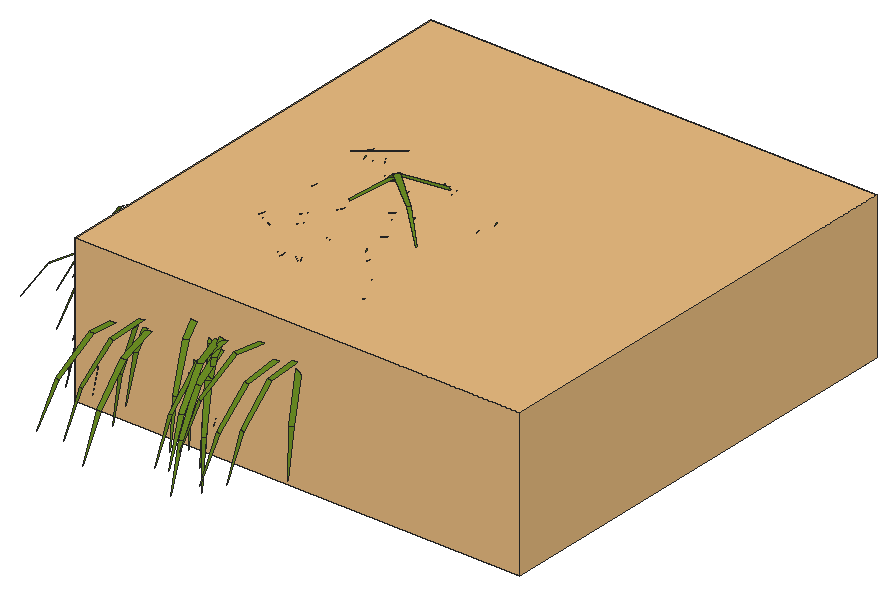
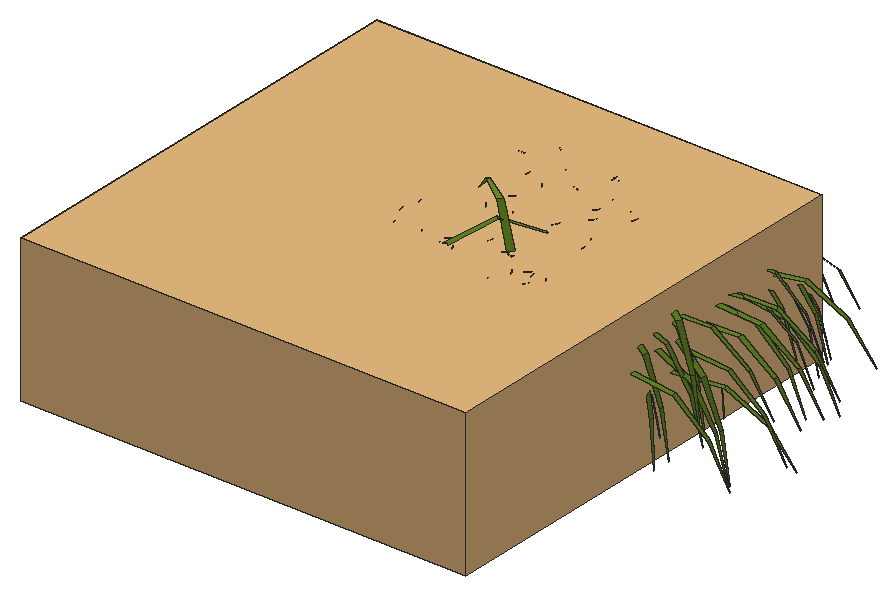
# SketchUp Ruby script. Lengths in inches.
U = 1.inch
M = Sketchup.active_model
def pt(a) = Geom::Point3d.new(a.map { |v| v * U })
def face(e, loops, mat)
  f = e.add_face(loops[0].map { |a| pt(a) })
  loops[1..].each { |l| e.add_face(l.map { |a| pt(a) }).erase! }
  f.material = f.back_material = mat if mat
  f
end
# faces: each face lists its corners as indices into pts; further lists are holes
def faces(e, pts, list, mat = nil) = list.each { |f| face(e, (f[0].is_a?(Array) ? f : [f]).map { |l| l.map { |i| pts[i] } }, mat) }
# xy, xz, yz: faces in a plane at the given z, y or x. An outline is a flat list of corners, or four numbers for a rectangle; further outlines are holes
def ring(l) = l.size == 4 ? [[l[0], l[1]], [l[2], l[1]], [l[2], l[3]], [l[0], l[3]]] : l.each_slice(2).to_a
def flat(e, list, mat, &to3) = list.each { |f| face(e, (f[0].is_a?(Array) ? f : [f]).map { |l| ring(l).map { |u, v| to3.(u, v) } }, mat) }
def xy(e, z, list, mat = nil) = flat(e, list, mat) { |x, y| [x, y, z] }
def xz(e, y, list, mat = nil) = flat(e, list, mat) { |x, z| [x, y, z] }
def yz(e, x, list, mat = nil) = flat(e, list, mat) { |y, z| [x, y, z] }
def lines(e, pts, list) = list.each { |a, b| e.add_line(pt(pts[a]), pt(pts[b])) }
# prism: a flat outline (further loops are holes) pulled along v
def prism(e, loops, v, mat = nil)
  f = face(e, loops, mat); d = Geom::Vector3d.new(v.map { |x| x * U })
  f.pushpull(f.normal.samedirection?(d) ? d.length : -d.length)
end
def box(e, o, s, mat = nil) = prism(e, [[o, [o[0] + s[0], o[1], o[2]], [o[0] + s[0], o[1] + s[1], o[2]], [o[0], o[1] + s[1], o[2]]]], [0, 0, s[2]], mat)
def at(x, y, z, deg = 0) = Geom::Transformation.translation(pt([x, y, z])) * Geom::Transformation.rotation(ORIGIN, Z_AXIS, deg.degrees)
def axes(o, x, y, z) = Geom::Transformation.new([*x, 0, *y, 0, *z, 0, *pt(o).to_a, 1])
def part(name) = M.definitions.add(name)
# library, detail: a bought-in or finely detailed component or shape, given as its bounding box
def library(name, o, s) = part(name).tap { |d| box(d.entities, o, s) }
def detail(e, o, s) = box(e.add_group.entities, o, s)
def put(e, d, t, mat = nil) = e.add_instance(d, t).tap { |i| i.material = mat if mat }
def group(e, t, mat = nil) = e.add_group.tap { |g| g.transformation = t; g.material = mat if mat }.entities
root = M.entities
M.materials.add("[0061_OliveDrab]").color = [107, 142, 35]
c1 = library("Group\#14",[0,0,0],[25.87,25.87,8.49])
xy(root,559.5,[[557.23,19.1,557.3125,19.22,557.42,19.375,555.26,20.87,555.11,20.65,555.44,20.4],[554.74,19.88,555.44,20.4,556.85,21.44,556.63,21.74,554.56,20.125]],"[0061_OliveDrab]")
p = [[545.64,15.02,552.99],[545.57,15.2,552.99],[544.4,14.6,550.72],[546.67,17.52,553.29],[546.64,17.74,553.29],[546.02,17.57,550.74],
  [559.23,3.76,553.36],[559.04,3.66,553.36],[559.37,3.27,550.78],[550.46,13.62,553.43],[550.58,13.78,553.43],[550.42,13.78,550.81],
  [546.54,17.27,553.32],[546.59,17.46,553.32],[545.875,17.57,550.79],[549.62,18.5,553.4],[549.64,18.7,553.4],[549.49,18.61,550.78],
  [549.27,7.625,553.47],[549.11,7.77,553.47],[548.89,7.36,550.89],[556.78,5.81,553.66],[556.58,5.75,553.66],[556.73,5.6,551.05],
  [549.94,13.07,553.6],[549.89,13.25,553.6],[549.78,13.125,550.98],[551.94,15.85,553.87],[551.74,15.9375,553.87],[551.81,15.8125,551.24],
  [554.33,2.23,553.68],[554.1,2.23,553.68],[554.23,1.0625,551.33],[559.01,2.33,553.77],[558.79,2.29,553.77],[559.03,1.45,551.29],
  [553.2,5.14,553.93],[553.01,5.21,553.93],[552.98,4.8,551.33],[549.55,6.52,553.9],[549.44,6.69,553.9],[549.03,6.29,551.34],
  [552.29,14.41,553.95],[552.5,14.41,553.95],[552.39,14.51,551.33],[552.61,3.01,553.92],[552.44,3.09,553.92],[552.1875,2.24,551.44],
  [546.33,10.34,553.83],[546.27,10.55,553.83],[545.41,10.19,551.37],[545.44,15.51,553.78],[545.43,15.7,553.78],[544.25,15.51,551.4375],
  [551.22,3.07,553.89],[551.02,3.13,553.89],[550.76,2.04,551.52],[551.1,6.38,554.05],[550.99,6.57,554.05],[550.64,6.25,551.47],
  [549.14,7.22,554.17],[549.07,7.43,554.17],[548.52,7.14,551.625],[559.6,9.88,554.26],[559.66,10.07,554.26],[559.54,10,551.64],
  [557.5,19.17,554.26],[557.67,19.31,554.26],[557.57,19.26,551.63],[556.19,20.15,554.26],[556.08,20.32,554.26],[556.11,20.22,551.63],
  [559.82,20.12,554.25],[559.73,20.29,554.25],[559.76,20.2,551.63],[558.89,4.19,554.32],[558.71,4.15,554.32],[558.9,3.71,551.74],
  [561.91,8.32,554.27],[561.82,8.15,554.27],[562.02,8.16,551.65],[556.73,9.18,554.3],[556.71,9.37,554.3],[556.54,9.25,551.68],
  [555.78,13.04,554.32],[555.73,12.83,554.32],[555.83,12.92,551.7],[556.41,13.68,554.29],[556.53,13.85,554.29],[556.4,13.82,551.67],
  [559.94,17.04,554.3125],[560.125,17,554.3125],[560.05,17.11,551.69],[561.04,19.43,554.28],[560.92,19.28,554.28],[561.02,19.33,551.66],
  [560.0625,20.97,554.35],[560.24,21.04,554.35],[560.125,21.08,551.72],[556.56,11.03,554.44],[556.39,11.12,554.44],[556.41,10.96,551.82],
  [559.97,11.54,554.41],[560.07,11.38,554.41],[560.11,11.52,551.78],[560.39,15.48,554.39],[560.26,15.65,554.39],[560.25,15.51,551.76],
  [556.46,16.08,554.42],[556.5625,16.27,554.42],[556.39,16.24,551.8],[553.86,16.69,554.46],[553.88,16.87,554.46],[553.72,16.79,551.84],
  [557.98,16.84,554.41],[557.81,16.92,554.41],[557.85,16.78,551.79],[545.54,19.45,554.18],[545.53,19.65,554.18],[544.37,19.49,551.83],
  [558.4,4.98,554.46],[558.22,4.88,554.46],[558.52,4.54,551.875],[560.53,6.55,554.48],[560.37,6.43,554.48],[560.64,6.24,551.875],
  [559.61,10.22,554.5],[559.45,10.33,554.5],[559.45,10.17,551.875],[546.625,12.32,554.43],[546.55,12.53,554.43],[545.8,12.16,551.9375],
  [561.8,13.99,554.47],[561.67,13.85,554.47],[561.84,13.82,551.85],[557.97,16.32,554.47],[557.83,16.46,554.47],[557.82,16.31,551.85],
  [562.625,18.43,554.48],[562.58,18.62,554.48],[562.44,18.48,551.86],[556.99,20.51,554.57],[557.05,20.31,554.57],[557.1875,20.45,551.95],
  [559.92,10.59,554.64],[559.9,10.4,554.64],[560.11,10.48,552.02],[559.9375,12.24,554.63],[560.1,12.1,554.63],[560.17,12.36,552.02],
  [554.9,13.12,554.57],[554.71,12.99,554.57],[554.9375,12.87,551.95],[558.4,14.875,554.62],[558.26,15.04,554.62],[558.18,14.84,552],
  [555.15,15.24,554.57],[555.29,15.41,554.57],[555.04,15.48,551.95],[560.81,15.64,554.58],[560.66,15.5,554.58],[560.85,15.45,551.96],
  [557.21,18.77,554.65],[557.08,18.61,554.65],[557.3,18.55,552.03],[558.02,2.76,554.58],[557.84,2.8,554.58],[557.74,1.89,552.12],
  [547.6875,10.47,554.62],[547.55,10.625,554.62],[547.03,10.03,552.11],[552.07,12.49,554.66],[552.18,12.65,554.66],[551.85,12.75,552.06],
  [562.51,14.52,554.73],[562.61,14.36,554.73],[562.77,14.58,552.12],[563.27,5.04,554.82],[563.07,4.98,554.82],[563.32,4.56,552.24],
  [552.86,6.9,554.79],[552.64,6.9375,554.79],[552.67,6.45,552.21],[558.29,10.5,554.77],[558.09,10.58,554.77],[558.1,10.3,552.16],
  [559.34,12.6,554.85],[559.47,12.43,554.85],[559.64,12.7,552.24],[558.39,12.87,554.83],[558.59,12.83,554.83],[558.55,13.13,552.22],
  [553.91,14.22,554.8],[553.78,14.38,554.8],[553.62,14.11,552.19],[556.83,14.35,554.77],[557.02,14.25,554.77],[557.05,14.54,552.16],
  [550.04,18.0625,554.77],[549.92,18.25,554.77],[549.67,17.96,552.17],[561.44,17.31,554.9],[561.41,17.5,554.9],[561.125,17.35,552.3],
  [548.29,19.41,554.87],[548.33,19.61,554.87],[547.78,19.62,552.3],[561.01,2.49,554.79],[560.8125,2.53,554.79],[560.71,1.48,552.39],
  [564.02,12.59,555],[563.99,12.39,555],[564.36,12.45,552.4],[547.89,17.8,555],[547.87,18,555],[547.27,17.82,552.45],
  [556.54,18.97,554.97],[556.57,19.15,554.97],[556.18,19.125,552.37],[548.49,8.71,555],[548.36,8.87,555],[547.83,8.32,552.48],
  [556.6875,16.66,555.09],[556.5,16.72,555.09],[556.48,16.33,552.49],[557.71,3.55,555.09],[557.53,3.49,555.09],[557.86,2.82,552.57],
  [558.35,6.21,555.17],[558.19,6.375,555.17],[557.91,5.94,552.59],[545.68,12.71,554.93],[545.66,12.91,554.93],[544.38,12.66,552.65],
  [548.23,16.91,555.15],[548.28,17.13,555.15],[547.67,17.15,552.59],[562.875,18.91,555.2],[563,18.74,555.2],[563.33,19.11,552.62],
  [553.98,5.35,555.24],[553.75,5.37,555.24],[553.79,4.73,552.69],[549.37,9.34,555.2],[549.29,9.53,555.2],[548.7,9.19,552.66],
  [545.9,11.21,555.1],[545.85,11.42,555.1],[544.6875,11.06,552.77],[562.35,2.61,555.29],[562.15,2.63,555.29],[562.13,1.66,552.85],
  [559.84,7.47,555.56],[559.67,7.6,555.56],[559.45,7.14,552.98],[560.34,10.8,555.6],[560.41,10.98,555.6],[559.87,11.08,553.03],
  [562.95,14.64,555.59],[563.14,14.63,555.59],[563.07,15.17,553.02],[547.51,15.76,554.69],[547.4,16.02,554.69],[558.14,9.88,555.62],
  [557.96,9.93,555.62],[557.91,9.38,553.05],[559.37,1.94,555.42],[559.16,1.88,555.42],[559.63,0.56,553.2],[553.71,9.72,555.8],
  [553.55,9.82,555.8],[553.31,9.26,553.24],[557.8,10.87,555.78],[557.66,11.03,555.78],[557.3125,10.58,553.22],[559.43,17.55,555.77],
  [559.28,17.72,555.77],[558.9375,17.25,553.21],[547.85,16.84,555.55],[547.93,17.11,555.55],[547.93,17.6,555.59],[547.9,17.91,555.59],
  [558.77,4.73,555.75],[558.5,4.59,555.75],[556.9,6.09,555.92],[556.72,6.03,555.92],[557.04,5.42,553.39],[550.7,13.38,556.03],
  [550.87,13.6,556.03],[545.22,14.9375,555.55],[545.24,15.16,555.55],[543.7,15.19,553.42],[550.01,18.42,555.99],[550.04,18.7,555.99],
  [549.98,8.34,555.9],[549.75,8.55,555.9],[546.02,8.74,555.63],[545.99,8.93,555.63],[544.54,8.625,553.47],[547.83,17.72,555.97],
  [547.92,17.89,555.97],[547.1,18.23,553.5],[559.81,19.26,556.08],[559.77,19.46,556.08],[559.12,19.22,553.54],[559.78,2.72,555.97],
  [559.57,2.79,555.97],[559.32,1.72,553.59],[555.83,8.69,556.12],[555.63,8.61,556.12],[555.99,8,553.59],[550.35,13.14,556.19],
  [550.28,13.4,556.19],[546.25,15.58,555.88],[546.22,15.78,555.88],[545.03,15.49,553.56],[560.9,19.07,556.1],[560.85,18.89,556.1],
  [561.51,18.8,553.56],[554.35,4.04,555.58],[554.03,4.04,555.58],[556.67,6.32,556.24],[556.39,6.23,556.24],[558.81,3.87,555.88],
  [558.5,3.82,555.88],[547.9,10.75,555.89],[547.8125,11.04,555.89],[547.37,15.625,555.56],[547.35,15.9,555.56],[553.25,4.44,556.03],
  [553.01,4.54,556.03],[551.85,4.82,555.74],[551.57,4.91,555.74],[553.54,5.99,556.39],[553.27,6.08,556.39],[550.5625,7.125,556.25],
  [550.4,7.375,556.25],[552.07,16.05,556.48],[551.79,16.17,556.48],[552.25,14.13,556.5625],[552.55,14.14,556.5625],[552.01,6.85,556.47],
  [551.87,7.11,556.47],[550.37,7.56,556.47],[550.28,7.85,556.47],[547.46,19.51,555.97],[547.44,19.8,555.97],[558.71,5.21,556.73],
  [558.45,5.16,556.73],[561.54,8.54,556.86],[561.42,8.3,556.86],[557.15,9.18,556.89],[557.125,9.46,556.89],[559.82,9.76,556.875],
  [559.92,10.03,556.875],[555.59,13.12,556.9375],[555.53,12.84,556.9375],[556.54,13.54,556.91],[556.71,13.78,556.91],[559.86,16.83,556.93],
  [560.12,16.78,556.93],[557.5,19.09,556.88],[557.74,19.3,556.88],[560.95,19.55,556.9],[560.79,19.33,556.9],[556.28,20.15,556.88],
  [556.12,20.4,556.88],[559.86,20.1,556.88],[559.74,20.34,556.88],[560.11,20.74,556.96],[560.36,20.83,556.96],[556.77,11.3125,557.04],
  [556.53,11.45,557.04],[559.7,11.41,557.01],[559.84,11.19,557.01],[548.12,12.78,556.54],[548.02,13.08,556.54],[560.63,15.62,557],
  [560.45,15.85,557],[556.74,15.87,557.02],[556.89,16.15,557.02],[558.14,17.09,557.02],[557.9,17.2,557.02],[557.97,5.88,556.89],
  [557.72,5.74,556.89],[560.12,7.16,557],[559.9,6.99,557],[559.85,10.52,557.1],[559.62,10.67,557.1],[561.55,14.26,557.07],
  [561.37,14.0625,557.07],[558.25,16.53,557.07],[558.04,16.74,557.07],[554.25,16.6,557.06],[554.28,16.86,557.06],[563.03,18.49,557.07],
  [562.96,18.76,557.07],[558.39,4.3125,556.67],[558.14,4.37,556.67],[559.41,10.67,557.21],[559.39,10.41,557.21],[548.84,11.45,556.76],
  [548.65,11.66,556.76],[559.56,11.82,557.19],[559.79,11.64,557.19],[554.63,13.6,557.13],[554.37,13.42,557.13],[555.53,14.87,557.14],
  [555.73,15.11,557.14],[558.8,15.15,557.2],[558.61,15.38,557.2],[560.53,15.99,557.17],[560.33,15.81,557.17],[556.85,19.14,557.22],
  [556.65,18.91,557.22],[556.54,20.4375,557.15],[556.62,20.15,557.15],[552.68,12.04,557.18],[552.83,12.27,557.18],[561.97,14.22,557.28],
  [562.12,14,557.28],[549.9,16.75,555.1],[549.77,17.06,555.1],[561.38,4.2,556.75],[561.11,4.25,556.75],[562.98,6.05,557.23],
  [562.7,5.95,557.23],[553.09,7.92,557.2],[552.78,7.97,557.2],[558.55,11.0625,557.32],[558.27,11.17,557.32],[558.77,12.21,557.38],
  [558.96,11.97,557.38],[558.2,12.22,557.37],[558.48,12.15,557.37],[556.49,13.8,557.32],[556.76,13.66,557.32],[554.45,14.62,557.34],
  [554.27,14.84,557.34],[550.78,18.47,557.26],[550.62,18.74,557.26],[547.67,12.89,556.64],[547.64,13.18,556.64],[562.16,17.4,557.43],
  [562.11,17.67,557.43],[549.41,19.14,557.23],[549.47,19.43,557.23],[549.64,9.57,557.19],[549.46,9.8,557.19],[563.23,12.72,557.5],
  [563.2,12.43,557.5],[549.16,17.93,557.3],[549.12,18.21,557.3],[557.32,18.78,557.47],[557.37,19.04,557.47],[557.27,4.94,557.27],
  [557.02,4.86,557.27],[547.82,11.57,556.85],[547.75,11.875,556.85],[549.4375,16.59,557.46],[549.51,16.9,557.46],[556.98,17.46,557.57],
  [556.71,17.54,557.57],[554.17,6.63,557.52],[553.86,6.66,557.52],[559.15,6.93,557.56],[558.93,7.16,557.56],[550.61,9.77,557.47],
  [550.51,10.04,557.47],[562.0625,18.37,557.64],[562.23,18.13,557.64],[562.6,4.3125,557.27],[562.33,4.35,557.27],[553.6,21.76,557.67],
  [553.71,21.92,557.67],[552.82,22.44,555.25],[558.87,3.98,557],[558.57,3.9,557],[553.16,18.74,557.74],[553.03,18.92,557.74],
  [552.21,18.16,555.36],[547.48,14.68,556.87],[547.5,15,556.87],[554.35,6.53,556.43],[553.96,6.52,556.43],[560.52,8.31,557.95],
  [560.28,8.49,557.95],[548.23,9.02,557.02],[548.19,9.29,557.02],[558.47,10.97,557.99],[558.22,11.03,557.99],[561.39,10.36,557.97],
  [561.49,10.625,557.97],[562.875,13.53,557.97],[563.14,13.52,557.97],[549.97,15.8,555.91],[549.9375,16.13,555.91],[550.07,16.16,556.76],
  [550.17,16.49,556.76],[550.18,17.79,556.93],[550.14,18.17,556.93],[552.7,7.26,556.22],[552.36,7.37,556.22],[557.8125,6.62,557.31],
  [557.49,6.45,557.31],[554.4,10.73,558.12],[554.17,10.88,558.12],[558.71,11.63,558.125],[558.51,11.85,558.125],[560.33,18.33,558.12],
  [560.11,18.56,558.12],[558.46,6.29,556.84],[558.08,6.23,556.84],[556.48,7.39,558.16],[556.23,7.3,558.16],[551.38,9.83,557.54],
  [551.1,10.08,557.54],[550.28,11.4,556.78],[550.18,11.75,556.78],[548.21,15.86,557.6],[548.17,16.125,557.6],[560.43,4.5,557.79],
  [560.14,4.6,557.79],[554.21,6.67,557.02],[553.92,6.8,557.02],[551.38,12.82,558.51],[551.58,13.09,558.51],[549.25,16.89,558.01],
  [549.38,17.12,558.01],[551.15,18.27,558.35],[551.18,18.625,558.35],[550.05,19.62,556.36],[550.03,19.97,556.36],[555.36,10,558.34],
  [555.07,9.89,558.34],[559.63,19.47,558.36],[559.55,19.21,558.36],[561.13,19.5,558.33],[561.07,19.79,558.33],[556.29,7.6875,558.44],
  [555.94,7.58,558.44],[552.44,8.32,557.64],[552.24,8.62,557.64],[551.49,13.43,558.54],[551.41,13.75,558.54],[554.22,7.83,558.14],
  [553.89,7.94,558.14],[553.84,7.84,558.07],[553.67,8.16,558.07],[552.59,8.22,557.69],[552.48,8.58,557.69],[550.49,13.56,557.34],
  [550.37,13.92,557.34],[552.35,16.61,559.03],[552.01,16.76,559.03],[550.25,13.16,557.04],[550.21,13.5,557.04],[552.22,13.36,559.07],
  [552.59,13.36,559.07],[550.07,14.4,556.59],[550.11,14.79,556.59],[558.94,6.7,557.61],[558.64,6.77,557.61],[558.3,7.27,558.3125],
  [557.98,7.2,558.3125],[561.9,6.65,557.53],[561.5625,6.71,557.53],[550.83,9.36,556.8125],[550.78,9.7,556.8125],[550.72,13.09,557.59],
  [550.48,13.35,557.59],[550.37,12.09,557.18],[550.29,12.46,557.18],[557.03,7.7,558.52],[556.72,7.54,558.52],[560.58,9.04,559.25],
  [560.4375,8.74,559.25],[558.125,9.26,559.33],[558.09,9.6,559.33],[560.46,9.51,559.41],[560.57,9.84,559.41],[555.04,13.28,559.5],
  [554.96,12.93,559.5],[556.85,13.29,559.5],[557.05,13.58,559.5],[559.73,16.33,559.5],[560.04,16.26,559.5],[557.59,18.9375,559.5],
  [557.67,19,559.5],[557.88,19.18,559.5],[560.67,19.8,559.5],[560.47,19.54,559.5],[556.4375,20.21,559.5],[556.24,20.52,559.5],
  [559.94,20.11,559.5],[559.8,20.4,559.5],[558.22,6.51,557.21],[557.86,6.42,557.21],[559.17,8.47,559.07],[558.89,8.26,559.07],
  [558.98,10.99,559.5],[559.15,10.71,559.5],[557.24,12.1,559.5],[556.96,12.26,559.5],[557.47,15.4375,559.5],[557.65,15.78,559.5],
  [561.26,16.08,559.5],[561.04,16.36,559.5],[558.52,17.84,559.5],[558.23,17.98,559.5],[560.3,20.11,559.5],[560.35,20.125,559.5],
  [560.61,20.22,559.5],[560.45,11.375,559.5],[560.17,11.5625,559.5],[553.9375,14.7,559.42],[553.61,14.48,559.42],[556.38,14.11,559.5],
  [556.63,14.41,559.5],[560.82,14.94,559.5],[560.61,14.7,559.5],[555.2,16.47,559.5],[555.23,16.78,559.5],[558.98,17.21,559.5],
  [558.72,17.47,559.5],[564,18.7,559.5],[563.92,19.03,559.5],[562.37,8.04,558.82],[562.02,7.93,558.82],[553.48,9.97,558.79],
  [553.11,10.04,558.79],[551.53,11.03,558.28],[551.32,11.3,558.28],[558.14,10.82,559.5],[558.12,10.67,559.5],[558.11,10.5,559.5],
  [558.76,10.86,559.5],[559.05,10.63,559.5],[554,11.15,559.26],[554.18,11.43,559.26],[559.8,15.93,559.5],[559.56,16.21,559.5],
  [559.74,16.9,559.5],[559.49,16.67,559.5],[551.57,18.68,558.64],[551.64,19.03,558.64],[555.89,20.01,559.5],[555.65,19.73,559.5],
  [555.4,20.17,559.5],[555.5,19.82,559.5],[562.95,6.85,557.82],[562.625,6.9,557.82],[556.5,7.28,558.19],[556.19,7.17,558.19],
  [559.11,12.41,559.5],[558.75,12.55,559.5],[555.77,12.53,559.5],[556.1,12.36,559.5],[560.78,13.49,559.5],[560.96,13.21,559.5],
  [555.62,15.54,559.5],[555.39,15.8125,559.5],[551.46,18.2,558.53],[551.41,18.54,558.53],[552.39,19.43,559.1],[552.19,19.75,559.1],
  [557.83,10.73,559.5],[558.18,10.66,559.5],[557.53,11.28,559.5],[557.76,10.99,559.5],[557.38,16.37,559.48],[557.22,16.5,559.48],
  [556.32,15.23,557.37],[563.75,17.66,559.5],[563.69,17.98,559.5],[554.48,8.95,558.72],[554.09,8.99,558.72],[552.77,10.55,558.74],
  [552.64,10.89,558.74],[561.55,12.93,559.5],[561.51,12.58,559.5],[551.68,16.0625,558.72],[551.76,16.44,558.72],[558.95,18.45,559.5],
  [559.01,18.76,559.5],[560.67,8.36,559.16],[560.4,8.63,559.16],[550.8,16.23,557.85],[550.74,16.5625,557.85],[560.55,17.31,559.5],
  [560.76,17.02,559.5],[557.53,19.15,559.5],[557.3125,19.22,559.5],[557.2,19.25,559.5],[554.74,19.88,559.5],[554.56,20.125,559.5],
  [555.11,20.65,559.5],[555.26,20.87,559.5],[561.31,6.96,558.04],[560.95,7.08,558.04],[561.83,9.98,559.49],[561.53,10.2,559.49],
  [563.42,9.5625,559.42],[563.54,9.89,559.42],[559.04,13.03,559.5],[558.74,13.11,559.5],[562.77,11.4,559.5],[563.09,11.39,559.5],
  [551.47,15.62,558.61],[551.63,15.91,558.61],[555.61,12.61,559.5],[555.33,12.78,559.5],[560.39,13.1,559.5],[560.15,13.37,559.5],
  [561.98,19.82,559.5],[561.72,20.1,559.5],[555.71,9.67,559.22],[555.4,9.56,559.22],[554.5,12.26,559.36],[554.15,12.12,559.36],
  [563.4375,19.97,559.5],[563.36,20.32,559.5],[557.36,20.15,559.5],[557.27,19.82,559.5],[561.32,16.04,560.75],[561.19,15.88,560.75],
  [562.84,14.71,559.06],[558.92,18.2,560.57],[558.68,18.39,560.57],[557.68,19.02,559.5],[557.46,18.74,559.5],[559.13,17.46,561.08],
  [559.31,17.69,561.08],[560.45,20.04,559.5],[560.16,20.27,559.5]]
faces(root,p,[[0,1,2],[3,4,5],[6,7,8],[9,10,11],[12,13,14],[15,16,17],[18,19,20],[21,22,23],
  [24,25,26],[27,28,29],[30,31,32],[33,34,35],[36,37,38],[39,40,41],[42,43,44],[45,46,47],
  [48,49,50],[51,52,53],[54,55,56],[57,58,59],[60,61,62],[63,64,65],[66,67,68],[69,70,71],
  [72,73,74],[75,76,77],[78,79,80],[81,82,83],[84,85,86],[87,88,89],[90,91,92],[93,94,95],
  [96,97,98],[99,100,101],[102,103,104],[105,106,107],[108,109,110],[111,112,113],[114,115,116],[117,118,119],
  [120,121,122],[123,124,125],[126,127,128],[129,130,131],[132,133,134],[135,136,137],[138,139,140],[141,142,143],
  [144,145,146],[147,148,149],[150,151,152],[153,154,155],[156,157,158],[159,160,161],[162,163,164],[165,166,167],
  [168,169,170],[171,172,173],[174,175,176],[177,178,179],[180,181,182],[183,184,185],[186,187,188],[189,190,191],
  [192,193,194],[195,196,197],[198,199,200],[201,202,203],[204,205,206],[207,208,209],[210,211,212],[213,214,215],
  [216,217,218],[219,220,221],[222,223,224],[225,226,227],[228,229,230],[231,232,233],[234,235,236],[237,238,239],
  [240,241,242],[243,244,245],[246,247,248],[249,250,251],[252,253,254],[255,256,257],[258,259,260],[261,262,1,0],
  [263,264,265],[266,267,268],[269,270,271],[272,273,274],[275,276,277],[278,279,13,12],[280,281,4,3],[282,283,7,6],
  [284,285,286],[287,288,10,9],[289,290,291],[292,293,16,15],[294,295,19,18],[296,297,298],[299,300,301],[302,303,304],
  [305,306,307],[308,309,310],[311,312,25,24],[313,314,315],[316,317,318],[319,320,31,30],[321,322,22,21],[323,324,34,33],
  [325,326,49,48],[327,328,52,51],[329,330,46,45],[331,332,55,54],[333,334,37,36],[335,336,40,39],[337,338,28,27],[339,340,43,42],
  [341,342,58,57],[343,344,61,60],[345,346,118,117],[347,348,76,75],[349,350,79,78],[351,352,82,81],[353,354,64,63],[355,356,85,84],
  [357,358,88,87],[359,360,91,90],[361,362,67,66],[363,364,94,93],[365,366,70,69],[367,368,73,72],[369,370,97,96],[371,372,100,99],
  [373,374,103,102],[375,376,130,129],[377,378,106,105],[379,380,109,108],[381,382,115,114],[383,384,121,120],[385,386,124,123],[387,388,127,126],
  [389,390,133,132],[391,392,136,135],[393,394,112,111],[395,396,139,138],[397,398,166,165],[399,400,145,144],[401,402,169,168],[403,404,148,147],
  [405,406,151,150],[407,408,157,156],[409,410,154,153],[411,412,160,159],[413,414,163,162],[415,416,142,141],[417,418,172,171],[419,420,175,174],
  [421,422,262,261],[423,424,208,207],[425,426,178,177],[427,428,181,180],[429,430,184,183],[431,432,187,186],[433,434,190,189],[435,436,196,195],
  [437,438,193,192],[439,440,199,198],[441,442,232,231],[443,444,202,201],[445,446,205,204],[447,448,220,219],[449,450,211,210],[451,452,214,213],
  [453,454,217,216],[455,456,226,225],[457,458,247,246],[459,460,235,234],[461,462,223,222],[463,464,241,240],[465,466,229,228],[467,468,244,243],
  [469,470,238,237],[471,472,250,249],[473,474,475],[476,477,267,266],[478,479,480],[481,482,290,289],[483,484,320,319],[485,486,253,252],
  [487,488,297,296],[489,490,264,263],[491,492,256,255],[493,494,259,258],[495,496,328,327],[497,498,279,278],[499,500,281,280],[501,502,332,331],
  [503,504,283,282],[505,506,270,269],[507,508,273,272],[509,510,276,275],[511,512,324,323],[513,514,285,284],[515,516,295,294],[517,518,326,325],
  [519,520,314,313],[521,522,306,305],[523,524,330,329],[525,526,288,287],[527,528,300,299],[529,530,293,292],[531,532,346,345],[533,534,309,308],
  [535,536,317,316],[537,538,303,302],[539,540,322,321],[541,542,336,335],[543,544,312,311],[545,546,334,333],[547,548,342,341],[549,550,344,343],
  [551,552,376,375],[553,554,338,337],[555,556,442,441],[557,558,340,339],[559,560,482,481],[561,562,398,397],[563,564,348,347],[565,566,424,423],
  [567,568,488,487],[569,570,402,401],[571,572,458,457],[573,574,384,383],[575,576,350,349],[577,578,352,351],[579,580,354,353],[581,582,356,355],
  [583,584,358,357],[585,586,360,359],[587,588,589,362,361],[590,591,364,363],[592,593,366,365],[594,595,368,367],[596,597,477,476],[598,599,386,385],
  [600,601,374,373],[602,603,372,371],[604,605,380,379],[606,607,378,377],[608,609,382,381],[610,611,612,370,369],[613,614,388,387],[615,616,406,405],
  [617,618,408,407],[619,620,390,389],[621,622,394,393],[623,624,392,391],[625,626,396,395],[627,628,426,425],[629,630,428,427],[631,632,448,447],
  [633,634,635,400,399],[636,637,404,403],[638,639,418,417],[640,641,410,409],[642,643,412,411],[644,645,446,445],[646,647,414,413],[648,649,416,415],
  [650,651,472,471],[652,653,456,455],[654,655,430,429],[656,657,436,435],[658,659,420,419],[660,661,438,437],[662,663,452,451],[664,665,440,439],
  [666,634,667,434,433],[668,669,432,431],[670,671,672],[673,674,444,443],[675,676,464,463],[677,678,468,467],[679,680,450,449],[681,682,460,459],
  [683,684,454,453],[685,686,466,465],[687,688,520,519],[689,690,470,469],[691,692,693,462,461],[694,695,479,478],[696,697,474,473],[698,699,522,521],
  [700,701,486,485],[702,703,492,491],[704,705,490,489],[706,707,494,493],[708,709,528,527],[710,711,506,505],[712,713,508,507],[714,715,510,509],
  [716,717,514,513],[718,719,534,533],[720,721,538,537],[722,723,536,535],[724,725,726],[727,728,671,670],[729,588,730,731,732],[733,611,734,728,727],
  [732,731,725,724]],"[0061_OliveDrab]")
put(root,c1,at(549.84,5.96,551.02))
